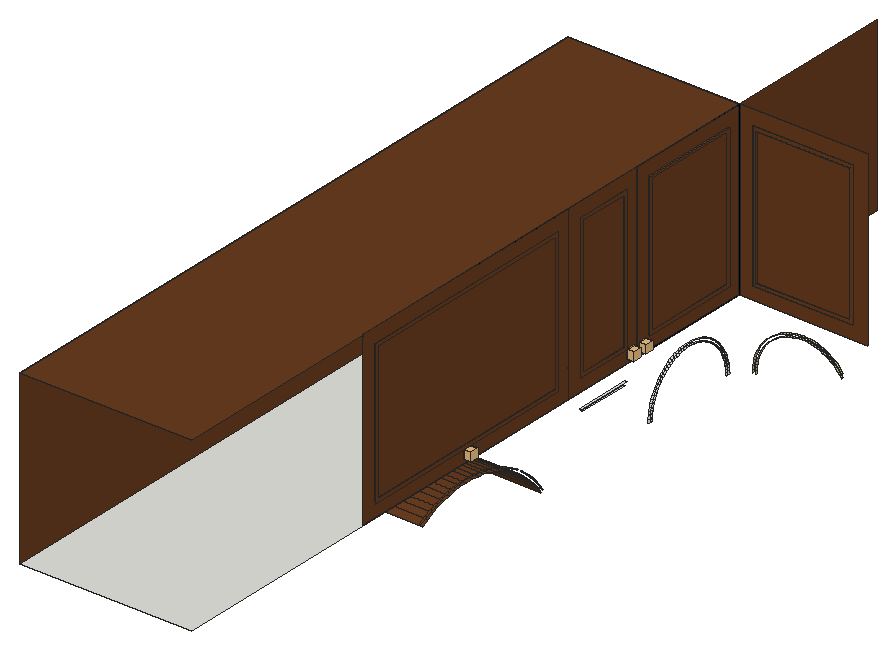
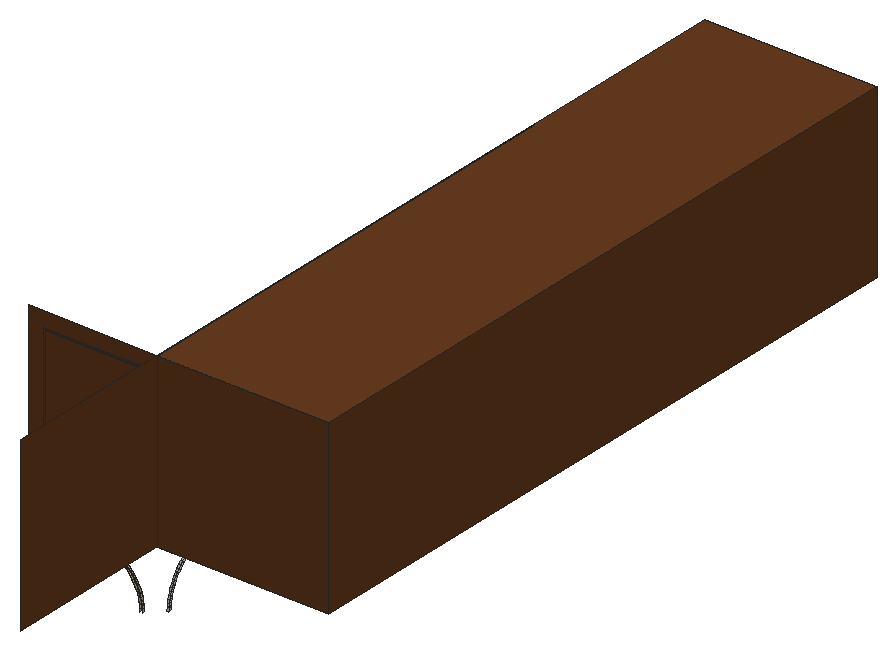
# SketchUp Ruby script. Lengths in inches.
U = 1.inch
M = Sketchup.active_model
def pt(a) = Geom::Point3d.new(a.map { |v| v * U })
def face(e, loops, mat)
  f = e.add_face(loops[0].map { |a| pt(a) })
  loops[1..].each { |l| e.add_face(l.map { |a| pt(a) }).erase! }
  f.material = f.back_material = mat if mat
  f
end
# faces: each face lists its corners as indices into pts; further lists are holes
def faces(e, pts, list, mat = nil) = list.each { |f| face(e, (f[0].is_a?(Array) ? f : [f]).map { |l| l.map { |i| pts[i] } }, mat) }
# xy, xz, yz: faces in a plane at the given z, y or x. An outline is a flat list of corners, or four numbers for a rectangle; further outlines are holes
def ring(l) = l.size == 4 ? [[l[0], l[1]], [l[2], l[1]], [l[2], l[3]], [l[0], l[3]]] : l.each_slice(2).to_a
def flat(e, list, mat, &to3) = list.each { |f| face(e, (f[0].is_a?(Array) ? f : [f]).map { |l| ring(l).map { |u, v| to3.(u, v) } }, mat) }
def xy(e, z, list, mat = nil) = flat(e, list, mat) { |x, y| [x, y, z] }
def xz(e, y, list, mat = nil) = flat(e, list, mat) { |x, z| [x, y, z] }
def yz(e, x, list, mat = nil) = flat(e, list, mat) { |y, z| [x, y, z] }
def lines(e, pts, list) = list.each { |a, b| e.add_line(pt(pts[a]), pt(pts[b])) }
# prism: a flat outline (further loops are holes) pulled along v
def prism(e, loops, v, mat = nil)
  f = face(e, loops, mat); d = Geom::Vector3d.new(v.map { |x| x * U })
  f.pushpull(f.normal.samedirection?(d) ? d.length : -d.length)
end
def box(e, o, s, mat = nil) = prism(e, [[o, [o[0] + s[0], o[1], o[2]], [o[0] + s[0], o[1] + s[1], o[2]], [o[0], o[1] + s[1], o[2]]]], [0, 0, s[2]], mat)
def at(x, y, z, deg = 0) = Geom::Transformation.translation(pt([x, y, z])) * Geom::Transformation.rotation(ORIGIN, Z_AXIS, deg.degrees)
def axes(o, x, y, z) = Geom::Transformation.new([*x, 0, *y, 0, *z, 0, *pt(o).to_a, 1])
def part(name) = M.definitions.add(name)
# library, detail: a bought-in or finely detailed component or shape, given as its bounding box
def library(name, o, s) = part(name).tap { |d| box(d.entities, o, s) }
def detail(e, o, s) = box(e.add_group.entities, o, s)
def put(e, d, t, mat = nil) = e.add_instance(d, t).tap { |i| i.material = mat if mat }
def group(e, t, mat = nil) = e.add_group.tap { |g| g.transformation = t; g.material = mat if mat }.entities
root = M.entities
M.materials.add("138_plaster painted wall texture-seamless").color = [214, 198, 153]
M.materials.add("[0137_Black]").color = [0, 0, 0]
M.materials.add("[Wood Veneer 01]").color = [104, 60, 32]
c1 = library("Group\#17",[0,0,0],[1.625,1.625,1.31])
xy(root,85.6,[[24,92.4,24.2,99.6]])
xy(root,86,[[24,92,24.2,100]])
xy(root,88,[[0,24,24,120]])
xy(root,90,[[24,56,24.2,88],[24,92,24.2,100],[24,104,24.2,118],[26,119.8,40,120]],"[Wood Veneer 01]")
xy(root,90.4,[[24,56.4,24.2,87.6],[24,92.4,24.2,99.6],[24,104.4,24.2,117.6],[26.4,119.8,39.6,120]],"[Wood Veneer 01]")
xy(root,109.6,[[24,56.4,24.2,87.6],[24,92.4,24.2,99.6],[24,104.4,24.2,117.6],[26.4,119.8,39.6,120]],"[Wood Veneer 01]")
xy(root,110,[[24,56,24.2,88],[24,92,24.2,100],[24,104,24.2,118],[26,119.8,40,120]],"[Wood Veneer 01]")
xy(root,112,[[0,24,24,120]],"[Wood Veneer 01]")
xz(root,87.6,[[24,90.4,24.2,109.6]],"[Wood Veneer 01]")
xz(root,88,[[24,90,24.2,110]],"[Wood Veneer 01]")
xz(root,92,[[24,90,24.2,110]],"[Wood Veneer 01]")
xz(root,92.4,[[24,90.4,24.2,109.6]],"[Wood Veneer 01]")
xz(root,99.6,[[24,90.4,24.2,109.6]],"[Wood Veneer 01]")
xz(root,100,[[24,90,24.2,110]],"[Wood Veneer 01]")
xz(root,104,[[24,90,24.2,110]],"[Wood Veneer 01]")
xz(root,104.4,[[24,90.4,24.2,109.6]],"[Wood Veneer 01]")
xz(root,117.6,[[24,90.4,24.2,109.6]])
xz(root,118,[[24,90,24.2,110]],"[Wood Veneer 01]")
xz(root,119.8,[[[26,90,40,110],[26.4,90.4,39.6,109.6]]],"[Wood Veneer 01]")
xz(root,120,[[0,88,24,112],[[24,88,42,112],[26,90,40,110]],[26.4,90.4,39.6,109.6]],"[Wood Veneer 01]")
yz(root,0,[[24,88,120,112]],"[Wood Veneer 01]")
yz(root,24,[[[54,88,90,112],[54.1,88.1,89.9,111.9]],[[90,88,102,112],[90.1,88.1,101.9,111.9]],[[102,88,120,112],[102.1,88.1,119.9,111.9]]],"[0137_Black]")
yz(root,24,[[120,88,144,112],[[54.1,88.1,89.9,111.9],[56,90,88,110]],[[90.1,88.1,101.9,111.9],[92,90,100,110]],[[102.1,88.1,119.9,111.9],[104,90,118,110]],[56.4,90.4,87.6,109.6],
  [92.4,90.4,99.6,109.6],[104.4,90.4,117.6,109.6]],"[Wood Veneer 01]")
yz(root,24.2,[[[56,90,88,110],[56.4,90.4,87.6,109.6]],[[92,90,100,110],[92.4,90.4,99.6,109.6]],[[104,90,118,110],[104.4,90.4,117.6,109.6]]],"[Wood Veneer 01]")
yz(root,26,[[119.8,90,120,110]],"[Wood Veneer 01]")
yz(root,26.4,[[119.8,90.4,120,109.6]],"[Wood Veneer 01]")
p = [[12,84.97,78.67],[24.2,84.97,78.67],[24.2,84.375,79.5],[12,84.375,79.5],[24,85.3,78.89],[24,84.69,79.74],
  [24.2,84.69,79.74],[24.2,85.3,78.89],[24,104.01,79.46],[24,104,79],[24.2,104,79],[24.2,104.01,79.46],
  [24,104.4,79],[24,104.41,79.43],[24.2,104.41,79.43],[24.2,104.4,79],[24,117.59,79.43],[24,117.6,79],
  [24.2,117.6,79],[24.2,117.59,79.43],[24,118,79],[24,117.99,79.46],[24.2,117.99,79.46],[24.2,118,79],
  [26.01,120,79.46],[26,120,79],[26,119.8,79],[26.01,119.8,79.46],[26.4,120,79],[26.41,120,79.43],
  [26.41,119.8,79.43],[26.4,119.8,79],[24,104.46,79.86],[24.2,104.46,79.86],[24,117.54,79.86],[24.2,117.54,79.86],
  [26.46,120,79.86],[26.46,119.8,79.86],[24.2,83.73,80.29],[12,83.73,80.29],[24,104.06,79.91],[24.2,104.06,79.91],
  [24,117.94,79.91],[24.2,117.94,79.91],[26.06,120,79.91],[26.06,119.8,79.91],[24,84.03,80.55],[24.2,84.03,80.55],
  [24,104.13,80.37],[24.2,104.13,80.37],[24,104.53,80.29],[24.2,104.53,80.29],[24,117.47,80.29],[24.2,117.47,80.29],
  [24,117.87,80.37],[24.2,117.87,80.37],[26.13,120,80.37],[26.13,119.8,80.37],[26.53,120,80.29],[26.53,119.8,80.29],
  [24.2,83.03,81.03],[12,83.03,81.03],[24,104.625,80.71],[24.2,104.625,80.71],[24,117.375,80.71],[24.2,117.375,80.71],
  [26.625,120,80.71],[26.625,119.8,80.71],[24,104.24,80.8125],[24.2,104.24,80.8125],[24,117.76,80.8125],[24.2,117.76,80.8125],
  [26.24,120,80.8125],[26.24,119.8,80.8125],[24,83.3125,81.3125],[24.2,83.3125,81.3125],[24,104.75,81.12],[24.2,104.75,81.12],
  [24,117.25,81.12],[24.2,117.25,81.12],[26.75,120,81.12],[26.75,119.8,81.12],[24,104.37,81.25],[24.2,104.37,81.25],
  [24,117.63,81.25],[24.2,117.63,81.25],[26.37,120,81.25],[26.37,119.8,81.25],[24.2,82.29,81.73],[12,82.29,81.73],
  [24,104.9,81.53],[24.2,104.9,81.53],[24,117.1,81.53],[24.2,117.1,81.53],[26.9,120,81.53],[26.9,119.8,81.53],
  [24,82.55,82.03],[24.2,82.55,82.03],[24,104.53,81.68],[24.2,104.53,81.68],[24,117.47,81.68],[24.2,117.47,81.68],
  [26.53,120,81.68],[26.53,119.8,81.68],[24,105.08,81.92],[24.2,105.08,81.92],[24,116.92,81.92],[24.2,116.92,81.92],
  [27.08,120,81.92],[27.08,119.8,81.92],[24.2,81.5,82.375],[12,81.5,82.375],[24,104.72,82.1],[24.2,104.72,82.1],
  [24,117.28,82.1],[24.2,117.28,82.1],[26.72,120,82.1],[26.72,119.8,82.1],[24,105.28,82.3],[24.2,105.28,82.3],
  [24,116.72,82.3],[24.2,116.72,82.3],[27.28,120,82.3],[27.28,119.8,82.3],[24,81.74,82.69],[24.2,81.74,82.69],
  [24,104.9375,82.5],[24.2,104.9375,82.5],[24,117.0625,82.5],[24.2,117.0625,82.5],[26.9375,120,82.5],[26.9375,119.8,82.5],
  [24,105.51,82.67],[24.2,105.51,82.67],[24,116.49,82.67],[24.2,116.49,82.67],[27.51,120,82.67],[27.51,119.8,82.67],
  [24.2,80.67,82.97],[12,80.67,82.97],[24,105.18,82.89],[24.2,105.18,82.89],[24,116.82,82.89],[24.2,116.82,82.89],
  [27.18,120,82.89],[27.18,119.8,82.89],[24,80.89,83.3],[24.2,80.89,83.3],[24,105.76,83.02],[24.2,105.76,83.02],
  [24,116.24,83.02],[24.2,116.24,83.02],[27.76,120,83.02],[27.76,119.8,83.02],[38.24,120,83.02],[38.49,120,82.67],
  [38.49,119.8,82.67],[38.24,119.8,83.02],[24,105.45,83.26],[24.2,105.45,83.26],[24,116.55,83.26],[24.2,116.55,83.26],
  [27.45,120,83.26],[27.45,119.8,83.26],[24.2,79.8,83.51],[12,79.8,83.51],[24,106.04,83.35],[24.2,106.04,83.35],
  [24,115.96,83.35],[24.2,115.96,83.35],[28.04,120,83.35],[28.04,119.8,83.35],[37.96,120,83.35],[37.96,119.8,83.35],
  [24,80,83.86],[24.2,80,83.86],[24,105.74,83.62],[24.2,105.74,83.62],[24,116.26,83.62],[24.2,116.26,83.62],
  [27.74,120,83.62],[27.74,119.8,83.62],[38.55,120,83.26],[38.26,120,83.62],[38.26,119.8,83.62],[38.55,119.8,83.26],
  [24,106.33,83.67],[24.2,106.33,83.67],[24,115.67,83.67],[24.2,115.67,83.67],[28.33,120,83.67],[28.33,119.8,83.67],
  [37.67,120,83.67],[37.67,119.8,83.67],[12,65.1,83.99],[24.2,65.1,83.99],[24.2,64.2,83.51],[12,64.2,83.51],
  [24.2,78.9,83.99],[12,78.9,83.99],[24,106.05,83.95],[24.2,106.05,83.95],[24,115.95,83.95],[24.2,115.95,83.95],
  [28.05,120,83.95],[28.05,119.8,83.95],[37.95,120,83.95],[37.95,119.8,83.95],[24,106.65,83.96],[24.2,106.65,83.96],
  [24,115.35,83.96],[24.2,115.35,83.96],[28.65,120,83.96],[28.65,119.8,83.96],[37.35,120,83.96],[37.35,119.8,83.96],
  [24,64.92,84.35],[24,64,83.86],[24.2,64,83.86],[24.2,64.92,84.35],[24,79.08,84.35],[24.2,79.08,84.35],
  [24,106.38,84.26],[24.2,106.38,84.26],[24,115.62,84.26],[24.2,115.62,84.26],[28.38,120,84.26],[28.38,119.8,84.26],
  [37.62,120,84.26],[37.62,119.8,84.26],[12,66.03,84.41],[24.2,66.03,84.41],[24.2,77.97,84.41],[12,77.97,84.41],
  [24,106.98,84.24],[24.2,106.98,84.24],[24,115.02,84.24],[24.2,115.02,84.24],[28.98,120,84.24],[28.98,119.8,84.24],
  [37.02,120,84.24],[37.02,119.8,84.24],[24,107.33,84.49],[24.2,107.33,84.49],[24,114.67,84.49],[24.2,114.67,84.49],
  [29.33,120,84.49],[29.33,119.8,84.49],[36.67,120,84.49],[36.67,119.8,84.49],[24,65.88,84.78],[24.2,65.88,84.78],
  [24,78.12,84.78],[24.2,78.12,84.78],[24,106.74,84.55],[24.2,106.74,84.55],[24,115.26,84.55],[24.2,115.26,84.55],
  [28.74,120,84.55],[28.74,119.8,84.55],[37.26,120,84.55],[37.26,119.8,84.55],[12,66.99,84.77],[24.2,66.99,84.77],
  [24.2,77.01,84.77],[12,77.01,84.77],[24,107.7,84.72],[24.2,107.7,84.72],[24,114.3,84.72],[24.2,114.3,84.72],
  [29.7,120,84.72],[29.7,119.8,84.72],[36.3,120,84.72],[36.3,119.8,84.72],[24,107.11,84.82],[24.2,107.11,84.82],
  [24,114.89,84.82],[24.2,114.89,84.82],[29.11,120,84.82],[29.11,119.8,84.82],[36.89,120,84.82],[36.89,119.8,84.82],
  [24,108.08,84.92],[24.2,108.08,84.92],[24,113.92,84.92],[24.2,113.92,84.92],[30.08,120,84.92],[30.08,119.8,84.92],
  [35.92,120,84.92],[35.92,119.8,84.92],[24,66.86,85.15],[24.2,66.86,85.15],[12,67.96,85.07],[24.2,67.96,85.07],
  [24.2,76.04,85.07],[12,76.04,85.07],[24,77.14,85.15],[24.2,77.14,85.15],[24,107.5,85.0625],[24.2,107.5,85.0625],
  [24,114.5,85.0625],[24.2,114.5,85.0625],[29.5,120,85.0625],[29.5,119.8,85.0625],[36.5,120,85.0625],[36.5,119.8,85.0625],
  [24,108.47,85.1],[24.2,108.47,85.1],[24,113.53,85.1],[24.2,113.53,85.1],[30.47,120,85.1],[30.47,119.8,85.1],
  [35.53,120,85.1],[35.53,119.8,85.1],[12,68.96,85.3],[24.2,68.96,85.3],[24.2,75.04,85.3],[12,75.04,85.3],
  [24,107.9,85.28],[24.2,107.9,85.28],[24,108.88,85.25],[24.2,108.88,85.25],[24,113.12,85.25],[24.2,113.12,85.25],
  [24,114.1,85.28],[24.2,114.1,85.28],[29.9,120,85.28],[29.9,119.8,85.28],[30.88,120,85.25],[30.88,119.8,85.25],
  [35.12,120,85.25],[35.12,119.8,85.25],[36.1,120,85.28],[36.1,119.8,85.28],[24,67.86,85.45],[24.2,67.86,85.45],
  [24,76.14,85.45],[24.2,76.14,85.45],[24,109.29,85.375],[24.2,109.29,85.375],[24,112.71,85.375],[24.2,112.71,85.375],
  [31.29,120,85.375],[31.29,119.8,85.375],[34.71,120,85.375],[34.71,119.8,85.375],[12,69.96,85.47],[24.2,69.96,85.47],
  [24.2,74.04,85.47],[12,74.04,85.47],[24,108.32,85.47],[24.2,108.32,85.47],[24,113.68,85.47],[24.2,113.68,85.47],
  [30.32,120,85.47],[30.32,119.8,85.47],[35.68,120,85.47],[35.68,119.8,85.47],[24,109.71,85.47],[24.2,109.71,85.47],
  [24,112.29,85.47],[24.2,112.29,85.47],[31.71,120,85.47],[31.71,119.8,85.47],[34.29,120,85.47],[34.29,119.8,85.47],
  [24,68.88,85.69],[24.2,68.88,85.69],[12,70.98,85.57],[24.2,70.98,85.57],[24.2,73.02,85.57],[12,73.02,85.57],
  [24,75.12,85.69],[24.2,75.12,85.69],[24,108.75,85.63],[24.2,108.75,85.63],[24,110.14,85.54],[24.2,110.14,85.54],
  [24,110.57,85.59],[24.2,110.57,85.59],[24,111.43,85.59],[24,111.86,85.54],[24.2,111.86,85.54],[24.2,111.43,85.59],
  [24,113.25,85.63],[24.2,113.25,85.63],[30.75,120,85.63],[30.75,119.8,85.63],[32.14,120,85.54],[32.14,119.8,85.54],
  [32.57,120,85.59],[32.57,119.8,85.59],[33.43,120,85.59],[33.86,120,85.54],[33.86,119.8,85.54],[33.43,119.8,85.59],
  [35.25,120,85.63],[35.25,119.8,85.63],[12,72,85.6],[24.2,72,85.6],[24,109.1875,85.76],[24.2,109.1875,85.76],
  [24,111,85.6],[24.2,111,85.6],[24,112.8125,85.76],[24.2,112.8125,85.76],[31.1875,120,85.76],[31.1875,119.8,85.76],
  [33,120,85.6],[33,119.8,85.6],[34.8125,120,85.76],[34.8125,119.8,85.76],[24,69.91,85.86],[24.2,69.91,85.86],
  [24,74.09,85.86],[24.2,74.09,85.86],[24,109.63,85.87],[24.2,109.63,85.87],[24,112.37,85.87],[24.2,112.37,85.87],
  [31.63,120,85.87],[31.63,119.8,85.87],[34.37,120,85.87],[34.37,119.8,85.87],[24,70.95,85.97],[24.2,70.95,85.97],
  [24,73.05,85.97],[24.2,73.05,85.97],[24,110.09,85.94],[24.2,110.09,85.94],[24,110.54,85.99],[24.2,110.54,85.99],
  [24,111.91,85.94],[24,111.46,85.99],[24.2,111.46,85.99],[24.2,111.91,85.94],[32.09,120,85.94],[32.09,119.8,85.94],
  [32.54,120,85.99],[32.54,119.8,85.99],[33.91,120,85.94],[33.46,120,85.99],[33.46,119.8,85.99],[33.91,119.8,85.94],
  [24,72,86],[24.2,72,86],[24,111,86],[24.2,111,86],[33,120,86],[33,119.8,86]]
faces(root,p,[[0,1,2,3],[4,5,6,7],[3,2,38,39],[5,46,47,6],[39,38,60,61],[46,74,75,47],[61,60,88,89],[74,96,97,75],
  [89,88,110,111],[96,124,125,97],[111,110,138,139],[124,146,147,125],[139,138,164,165],[146,174,175,147],[194,195,196,197],[165,164,198,199],
  [216,217,218,219],[174,220,221,175],[230,231,195,194],[199,198,232,233],[250,216,219,251],[220,252,253,221],[262,263,231,230],[233,232,264,265],
  [290,250,251,291],[292,293,263,262],[265,264,294,295],[252,296,297,253],[314,315,293,292],[295,294,316,317],[334,290,291,335],[296,336,337,297],
  [346,347,315,314],[317,316,348,349],[366,334,335,367],[368,369,347,346],[349,348,370,371],[336,372,373,337],[398,399,369,368],[371,370,399,398],
  [412,366,367,413],[372,414,415,373],[424,412,413,425],[414,426,427,415],[444,424,425,445],[426,444,445,427]],"[Wood Veneer 01]")
faces(root,p,[[8,9,10,11],[12,13,14,15],[16,17,18,19],[20,21,22,23],[13,32,33,14],[34,16,19,35],[40,8,11,41],[21,42,43,22],
  [48,40,41,49],[32,50,51,33],[52,34,35,53],[42,54,55,43],[50,62,63,51],[64,52,53,65],[68,48,49,69],[54,70,71,55],
  [62,76,77,63],[78,64,65,79],[82,68,69,83],[70,84,85,71],[76,90,91,77],[92,78,79,93],[98,82,83,99],[84,100,101,85],
  [90,104,105,91],[106,92,93,107],[112,98,99,113],[100,114,115,101],[104,118,119,105],[120,106,107,121],[126,112,113,127],[114,128,129,115],
  [118,132,133,119],[134,120,121,135],[140,126,127,141],[128,142,143,129],[132,148,149,133],[150,134,135,151],[158,140,141,159],[142,160,161,143],
  [148,166,167,149],[168,150,151,169],[176,158,159,177],[160,178,179,161],[166,186,187,167],[188,168,169,189],[200,176,177,201],[178,202,203,179],
  [186,208,209,187],[210,188,189,211],[222,200,201,223],[202,224,225,203],[208,234,235,209],[236,210,211,237],[234,242,243,235],[244,236,237,245],
  [254,222,223,255],[224,256,257,225],[242,266,267,243],[268,244,245,269],[274,254,255,275],[256,276,277,257],[266,282,283,267],[284,268,269,285],
  [298,274,275,299],[276,300,301,277],[282,306,307,283],[308,284,285,309],[318,298,299,319],[306,320,321,307],[322,308,309,323],[300,324,325,301],
  [320,338,339,321],[340,322,323,341],[350,318,319,351],[324,352,353,325],[338,358,359,339],[360,340,341,361],[374,350,351,375],[358,376,377,359],
  [376,378,379,377],[380,381,382,383],[381,360,361,382],[352,384,385,353],[400,374,375,401],[378,402,403,379],[402,380,383,403],[384,404,405,385],
  [416,400,401,417],[404,418,419,405],[428,416,417,429],[430,428,429,431],[432,433,434,435],[418,432,435,419],[446,430,431,447],[433,446,447,434]])
faces(root,p,[[24,25,26,27],[28,29,30,31],[29,36,37,30],[44,24,27,45],[56,44,45,57],[36,58,59,37],[58,66,67,59],[72,56,57,73],
  [66,80,81,67],[86,72,73,87],[80,94,95,81],[102,86,87,103],[94,108,109,95],[116,102,103,117],[108,122,123,109],[130,116,117,131],
  [122,136,137,123],[144,130,131,145],[136,152,153,137],[154,155,156,157],[162,144,145,163],[152,170,171,153],[172,154,157,173],[180,162,163,181],
  [182,183,184,185],[170,190,191,171],[192,172,173,193],[204,180,181,205],[183,206,207,184],[190,212,213,191],[214,192,193,215],[226,204,205,227],
  [206,228,229,207],[212,238,239,213],[240,214,215,241],[238,246,247,239],[248,240,241,249],[258,226,227,259],[228,260,261,229],[246,270,271,247],
  [272,248,249,273],[278,258,259,279],[260,280,281,261],[270,286,287,271],[288,272,273,289],[302,278,279,303],[280,304,305,281],[286,310,311,287],
  [312,288,289,313],[326,302,303,327],[310,328,329,311],[330,312,313,331],[304,332,333,305],[328,342,343,329],[344,330,331,345],[354,326,327,355],
  [332,356,357,333],[342,362,363,343],[364,344,345,365],[386,354,355,387],[362,388,389,363],[388,390,391,389],[392,393,394,395],[393,364,365,394],
  [356,396,397,357],[406,386,387,407],[390,408,409,391],[408,392,395,409],[396,410,411,397],[420,406,407,421],[410,422,423,411],[436,420,421,437],
  [438,436,437,439],[440,441,442,443],[422,440,443,423],[448,438,439,449],[441,448,449,442]],"138_plaster painted wall texture-seamless")
put(root,c1,axes([24,72.875,89.82],[0,-0.74,0],[0,0,-0.74],[0.74,0,0]),"[Wood Veneer 01]")
put(root,c1,axes([24,101.5625,89.82],[0,-0.74,0],[0,0,-0.74],[0.74,0,0]),"[Wood Veneer 01]")
put(root,c1,axes([24,103.625,89.82],[0,-0.74,0],[0,0,-0.74],[0.74,0,0]),"[Wood Veneer 01]")
